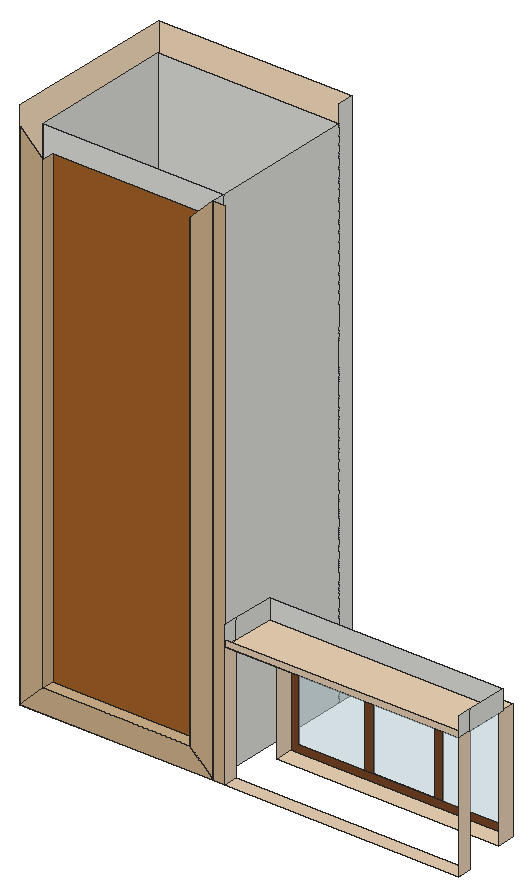
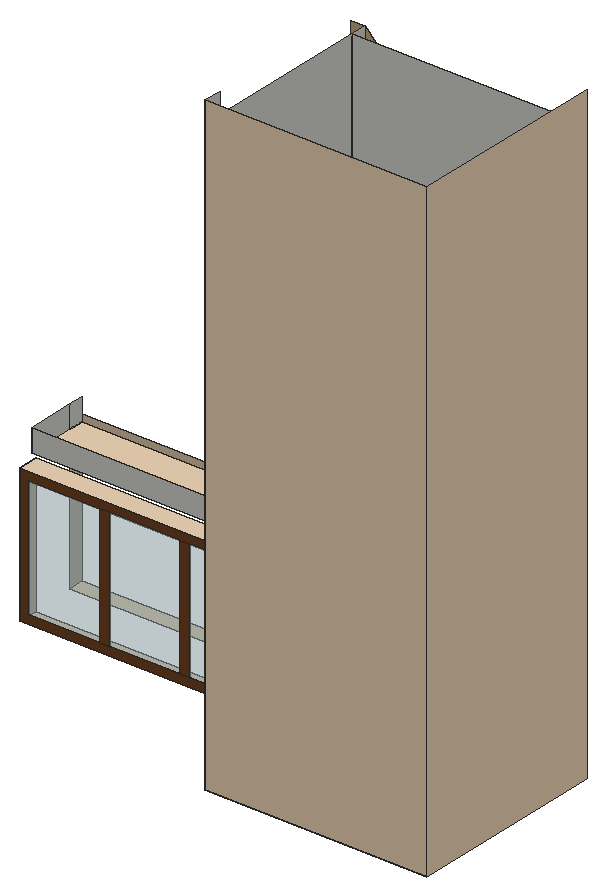
# SketchUp Ruby script. Lengths in inches.
U = 1.inch
M = Sketchup.active_model
def pt(a) = Geom::Point3d.new(a.map { |v| v * U })
def face(e, loops, mat)
  f = e.add_face(loops[0].map { |a| pt(a) })
  loops[1..].each { |l| e.add_face(l.map { |a| pt(a) }).erase! }
  f.material = f.back_material = mat if mat
  f
end
# faces: each face lists its corners as indices into pts; further lists are holes
def faces(e, pts, list, mat = nil) = list.each { |f| face(e, (f[0].is_a?(Array) ? f : [f]).map { |l| l.map { |i| pts[i] } }, mat) }
# xy, xz, yz: faces in a plane at the given z, y or x. An outline is a flat list of corners, or four numbers for a rectangle; further outlines are holes
def ring(l) = l.size == 4 ? [[l[0], l[1]], [l[2], l[1]], [l[2], l[3]], [l[0], l[3]]] : l.each_slice(2).to_a
def flat(e, list, mat, &to3) = list.each { |f| face(e, (f[0].is_a?(Array) ? f : [f]).map { |l| ring(l).map { |u, v| to3.(u, v) } }, mat) }
def xy(e, z, list, mat = nil) = flat(e, list, mat) { |x, y| [x, y, z] }
def xz(e, y, list, mat = nil) = flat(e, list, mat) { |x, z| [x, y, z] }
def yz(e, x, list, mat = nil) = flat(e, list, mat) { |y, z| [x, y, z] }
def lines(e, pts, list) = list.each { |a, b| e.add_line(pt(pts[a]), pt(pts[b])) }
# prism: a flat outline (further loops are holes) pulled along v
def prism(e, loops, v, mat = nil)
  f = face(e, loops, mat); d = Geom::Vector3d.new(v.map { |x| x * U })
  f.pushpull(f.normal.samedirection?(d) ? d.length : -d.length)
end
def box(e, o, s, mat = nil) = prism(e, [[o, [o[0] + s[0], o[1], o[2]], [o[0] + s[0], o[1] + s[1], o[2]], [o[0], o[1] + s[1], o[2]]]], [0, 0, s[2]], mat)
def at(x, y, z, deg = 0) = Geom::Transformation.translation(pt([x, y, z])) * Geom::Transformation.rotation(ORIGIN, Z_AXIS, deg.degrees)
def axes(o, x, y, z) = Geom::Transformation.new([*x, 0, *y, 0, *z, 0, *pt(o).to_a, 1])
def part(name) = M.definitions.add(name)
# library, detail: a bought-in or finely detailed component or shape, given as its bounding box
def library(name, o, s) = part(name).tap { |d| box(d.entities, o, s) }
def detail(e, o, s) = box(e.add_group.entities, o, s)
def put(e, d, t, mat = nil) = e.add_instance(d, t).tap { |i| i.material = mat if mat }
def group(e, t, mat = nil) = e.add_group.tap { |g| g.transformation = t; g.material = mat if mat }.entities
root = M.entities
M.materials.add("[0012_Bisque]").color = [234, 209, 180]
M.materials.add("[0012_Bisque]1").color = [237, 212, 182]
M.materials.add("[0012_Bisque]3").color = [255, 228, 196]
M.materials.add("[0035_Tan]").color = [210, 180, 140]
M.materials.add("[Translucent Glass Safety]1").color = [204, 235, 244]
M.materials["[Translucent Glass Safety]1"].alpha = 0.5
M.materials.add("[Wood Bamboo]").color = [165, 98, 40]
M.materials.add("[Wood Veneer 01]").color = [120, 70, 37]
xy(root,109.8125,[[65.97,364.57,65.97,487.49,202.72,487.49,202.72,476.36,74.5,476.36,74.5,374.1875,202.72,374.1875,202.72,364.57],[74.5,374.1875,202.72,476.36]])
xy(root,109.8125,[[211.5,364.57,376.86,374.19]],"[0012_Bisque]")
xy(root,111.1,[[216.9,403.76,374.03,416.01]],"[0012_Bisque]1")
xy(root,126.03,[[82.19,364.57,186.51,373.01]],"[0035_Tan]")
xy(root,196.03,[[216.9,403.76,374.03,416.01]],"[0012_Bisque]1")
xy(root,197.75,[[211.5,364.57,376.86,403.76]],"[0012_Bisque]1")
xz(root,364.57,[[211.5,197.75,376.86,201.93]],"[0012_Bisque]")
xz(root,364.57,[[65.97,109.8125,202.72,109.8125,186.51,126.03,82.19,126.03],[65.97,109.8125,82.19,126.03,82.19,461.22,65.97,477.4375],[202.72,109.8125,202.72,477.4375,186.51,461.22,186.51,126.03],[202.72,109.8125,211.5,477.4375]],"[0035_Tan]")
xz(root,373.01,[[82.19,126.03,186.51,461.22]],"[Wood Bamboo]")
xz(root,374.1875,[[74.5,109.8125,202.72,477.4375]])
xz(root,403.76,[[211.5,197.75,376.86,211.6875]])
xz(root,416.01,[[222.25,116.44,269.31,190.6875],[275.53,116.44,318.68,190.6875],[324.91,116.44,368.68,190.6875]],"[Translucent Glass Safety]1")
xz(root,416.01,[[[216.9,111.1,374.03,196.03],[222.25,116.44,368.68,190.6875]],[269.31,116.44,275.53,190.6875],[318.68,116.44,324.91,190.6875]],"[Wood Veneer 01]")
xz(root,476.36,[[74.5,109.8125,202.72,477.4375]])
xz(root,487.49,[[65.97,109.8125,202.72,490.375]],"[0012_Bisque]3")
yz(root,65.97,[[364.57,109.8125,487.49,490.375]],"[0012_Bisque]3")
yz(root,74.5,[[374.1875,109.8125,476.36,477.4375]])
yz(root,82.19,[[364.57,126.03,373.01,461.22]],"[0035_Tan]")
yz(root,186.51,[[364.57,126.03,373.01,461.22]],"[0035_Tan]")
yz(root,202.72,[[364.57,109.8125,374.1875,477.4375],[374.1875,109.8125,476.36,477.4375],[476.36,109.8125,487.49,490.375]])
yz(root,211.5,[[364.57,197.75,374.19,211.6875],[374.19,197.75,403.76,211.6875]])
yz(root,211.5,[[364.57,109.8125,374.19,197.75]],"[0012_Bisque]1")
yz(root,216.9,[[403.76,111.1,416.01,196.03]],"[0012_Bisque]1")
yz(root,374.03,[[403.76,111.1,416.01,196.03]],"[0012_Bisque]1")
yz(root,376.86,[[364.57,197.75,374.19,211.6875],[374.19,197.75,403.76,211.6875]])
yz(root,376.86,[[364.57,109.8125,374.19,197.75]],"[0012_Bisque]1")
